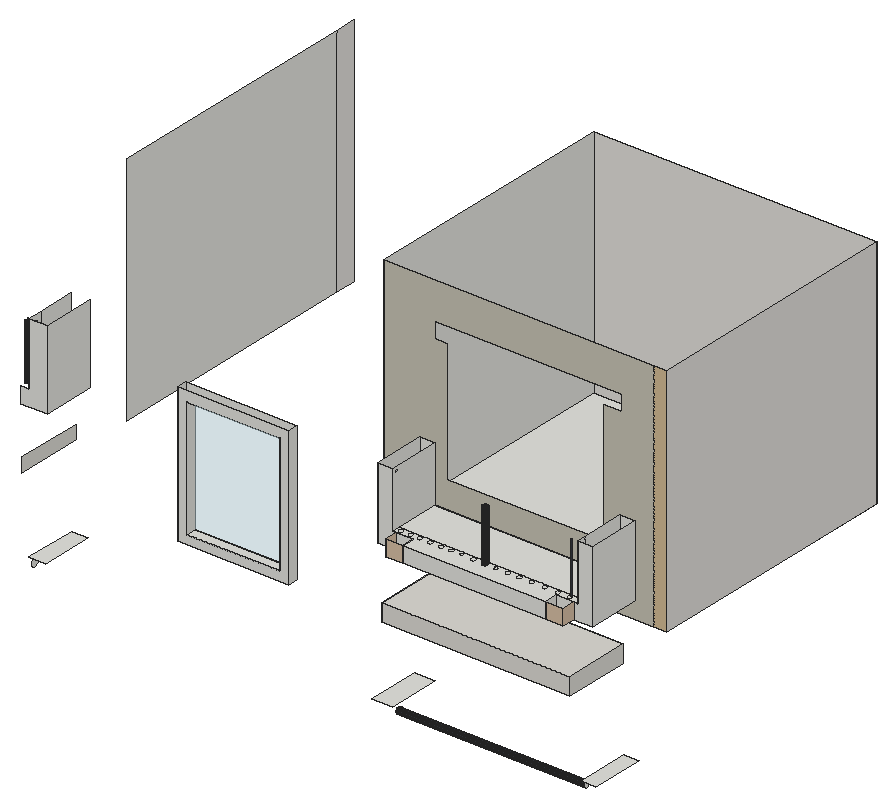
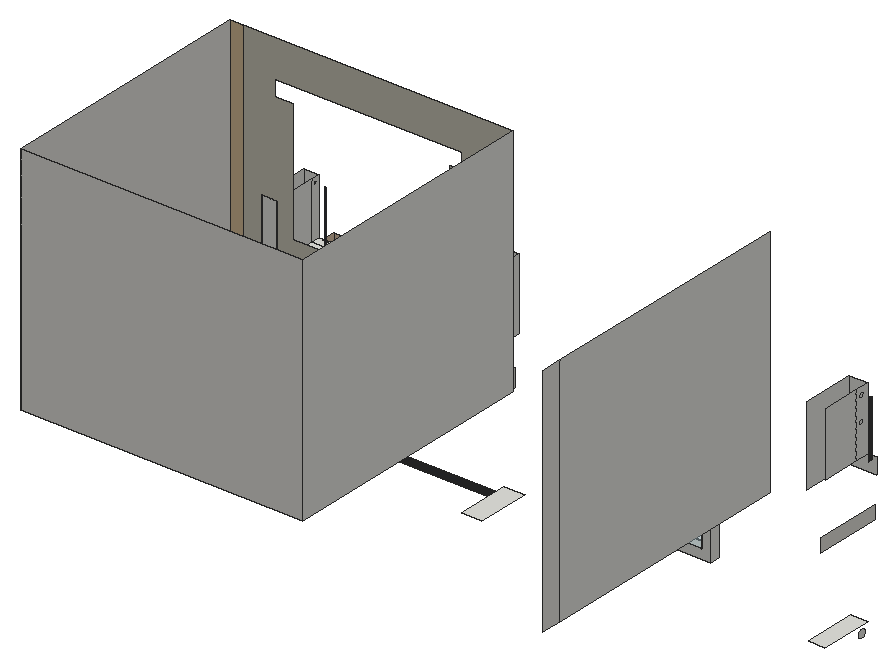
# SketchUp Ruby script. Lengths in inches.
U = 1.inch
M = Sketchup.active_model
def pt(a) = Geom::Point3d.new(a.map { |v| v * U })
def face(e, loops, mat)
  f = e.add_face(loops[0].map { |a| pt(a) })
  loops[1..].each { |l| e.add_face(l.map { |a| pt(a) }).erase! }
  f.material = f.back_material = mat if mat
  f
end
# faces: each face lists its corners as indices into pts; further lists are holes
def faces(e, pts, list, mat = nil) = list.each { |f| face(e, (f[0].is_a?(Array) ? f : [f]).map { |l| l.map { |i| pts[i] } }, mat) }
# xy, xz, yz: faces in a plane at the given z, y or x. An outline is a flat list of corners, or four numbers for a rectangle; further outlines are holes
def ring(l) = l.size == 4 ? [[l[0], l[1]], [l[2], l[1]], [l[2], l[3]], [l[0], l[3]]] : l.each_slice(2).to_a
def flat(e, list, mat, &to3) = list.each { |f| face(e, (f[0].is_a?(Array) ? f : [f]).map { |l| ring(l).map { |u, v| to3.(u, v) } }, mat) }
def xy(e, z, list, mat = nil) = flat(e, list, mat) { |x, y| [x, y, z] }
def xz(e, y, list, mat = nil) = flat(e, list, mat) { |x, z| [x, y, z] }
def yz(e, x, list, mat = nil) = flat(e, list, mat) { |y, z| [x, y, z] }
def lines(e, pts, list) = list.each { |a, b| e.add_line(pt(pts[a]), pt(pts[b])) }
# prism: a flat outline (further loops are holes) pulled along v
def prism(e, loops, v, mat = nil)
  f = face(e, loops, mat); d = Geom::Vector3d.new(v.map { |x| x * U })
  f.pushpull(f.normal.samedirection?(d) ? d.length : -d.length)
end
def box(e, o, s, mat = nil) = prism(e, [[o, [o[0] + s[0], o[1], o[2]], [o[0] + s[0], o[1] + s[1], o[2]], [o[0], o[1] + s[1], o[2]]]], [0, 0, s[2]], mat)
def at(x, y, z, deg = 0) = Geom::Transformation.translation(pt([x, y, z])) * Geom::Transformation.rotation(ORIGIN, Z_AXIS, deg.degrees)
def axes(o, x, y, z) = Geom::Transformation.new([*x, 0, *y, 0, *z, 0, *pt(o).to_a, 1])
def part(name) = M.definitions.add(name)
# library, detail: a bought-in or finely detailed component or shape, given as its bounding box
def library(name, o, s) = part(name).tap { |d| box(d.entities, o, s) }
def detail(e, o, s) = box(e.add_group.entities, o, s)
def put(e, d, t, mat = nil) = e.add_instance(d, t).tap { |i| i.material = mat if mat }
def group(e, t, mat = nil) = e.add_group.tap { |g| g.transformation = t; g.material = mat if mat }.entities
root = M.entities
M.materials.add("[Color M07]").color = [58, 58, 58]
M.materials.add("[Formica Beige]").color = [211, 187, 149]
M.materials.add("[Formica Graystone]").color = [198, 194, 180]
M.materials.add("[Formica Laminate Dark]").color = [50, 53, 60]
M.materials.add("[Formica Laminate Light]").color = [213, 189, 164]
M.materials.add("[Quartz Light Brown]").color = [199, 184, 152]
M.materials.add("[Terrazzo Tile Accent]").color = [224, 221, 217]
M.materials.add("[Terrazzo Tile Light]").color = [219, 217, 210]
M.materials.add("[Translucent Glass Safety]").color = [204, 235, 244]
M.materials["[Translucent Glass Safety]"].alpha = 0.5
xy(root,296.55,[[376.7,92.22,376.96,92.25,377.2,92.35,377.41,92.51,377.57,92.72,377.67,92.96,377.7,93.22,377.67,93.48,377.57,93.72,377.41,93.93,377.2,94.09,376.96,94.1875,376.7,94.22,376.44,94.1875,376.2,94.09,375.99,93.93,375.83,93.72,375.73,93.48,375.7,93.22,375.73,92.96,375.83,92.72,375.99,92.51,376.2,92.35,376.44,92.25]])
xy(root,296.68,[[303.57,92.22,303.83,92.25,304.07,92.35,304.28,92.51,304.44,92.72,304.54,92.96,304.57,93.22,304.54,93.48,304.44,93.72,304.28,93.93,304.07,94.09,303.83,94.1875,303.57,94.22,303.32,94.1875,303.07,94.09,302.87,93.93,302.71,93.72,302.61,93.48,302.57,93.22,302.61,92.96,302.71,92.72,302.87,92.51,303.07,92.35,303.32,92.25],[370.57,92.22,370.83,92.25,371.07,92.35,371.28,92.51,371.44,92.72,371.54,92.96,371.57,93.22,371.54,93.48,371.44,93.72,371.28,93.93,371.07,94.09,370.83,94.1875,370.57,94.22,370.32,94.1875,370.07,94.09,369.87,93.93,369.71,93.72,369.61,93.48,369.57,93.22,369.61,92.96,369.71,92.72,369.87,92.51,370.07,92.35,370.32,92.25]])
xy(root,296.93,[[352.2,92.22,352.46,92.25,352.7,92.35,352.91,92.51,353.07,92.72,353.17,92.96,353.2,93.22,353.17,93.48,353.07,93.72,352.91,93.93,352.7,94.09,352.46,94.1875,352.2,94.22,351.94,94.1875,351.7,94.09,351.49,93.93,351.33,93.72,351.23,93.48,351.2,93.22,351.23,92.96,351.33,92.72,351.49,92.51,351.7,92.35,351.94,92.25]])
xy(root,297.05,[[298.07,92.22,298.33,92.25,298.57,92.35,298.78,92.51,298.94,92.72,299.04,92.96,299.07,93.22,299.04,93.48,298.94,93.72,298.78,93.93,298.57,94.09,298.33,94.1875,298.07,94.22,297.82,94.1875,297.57,94.09,297.37,93.93,297.21,93.72,297.11,93.48,297.07,93.22,297.11,92.96,297.21,92.72,297.37,92.51,297.57,92.35,297.82,92.25],[323.57,92.22,323.83,92.25,324.07,92.35,324.28,92.51,324.44,92.72,324.54,92.96,324.57,93.22,324.54,93.48,324.44,93.72,324.28,93.93,324.07,94.09,323.83,94.1875,323.57,94.22,323.32,94.1875,323.07,94.09,322.87,93.93,322.71,93.72,322.61,93.48,322.57,93.22,322.61,92.96,322.71,92.72,322.87,92.51,323.07,92.35,323.32,92.25]])
xy(root,297.11,[[337.23,91.64,337.68,91.7,338.11,91.875,338.47,92.15,338.75,92.51,338.92,92.9375,338.98,93.39,338.92,93.84,338.75,94.26,338.47,94.625,338.11,94.9,337.68,95.08,337.23,95.14,336.78,95.08,336.36,94.9,335.99,94.625,335.72,94.26,335.54,93.84,335.48,93.39,335.54,92.9375,335.72,92.51,335.99,92.15,336.36,91.875,336.78,91.7]],"[Formica Laminate Dark]")
xy(root,297.18,[[329.95,92.22,330.21,92.25,330.45,92.35,330.66,92.51,330.82,92.72,330.92,92.96,330.95,93.22,330.92,93.48,330.82,93.72,330.66,93.93,330.45,94.09,330.21,94.1875,329.95,94.22,329.69,94.1875,329.45,94.09,329.24,93.93,329.08,93.72,328.98,93.48,328.95,93.22,328.98,92.96,329.08,92.72,329.24,92.51,329.45,92.35,329.69,92.25]])
xy(root,297.44,[[316.7,92.22,316.96,92.25,317.2,92.35,317.41,92.51,317.57,92.72,317.67,92.96,317.7,93.22,317.67,93.48,317.57,93.72,317.41,93.93,317.2,94.09,316.96,94.1875,316.7,94.22,316.44,94.1875,316.2,94.09,315.99,93.93,315.83,93.72,315.73,93.48,315.7,93.22,315.73,92.96,315.83,92.72,315.99,92.51,316.2,92.35,316.44,92.25]])
xy(root,297.55,[[345.7,92.22,345.96,92.25,346.2,92.35,346.41,92.51,346.57,92.72,346.67,92.96,346.7,93.22,346.67,93.48,346.57,93.72,346.41,93.93,346.2,94.09,345.96,94.1875,345.7,94.22,345.44,94.1875,345.2,94.09,344.99,93.93,344.83,93.72,344.73,93.48,344.7,93.22,344.73,92.96,344.83,92.72,344.99,92.51,345.2,92.35,345.44,92.25]])
xy(root,297.74,[[310.2,92.22,310.46,92.25,310.7,92.35,310.91,92.51,311.07,92.72,311.17,92.96,311.2,93.22,311.17,93.48,311.07,93.72,310.91,93.93,310.7,94.09,310.55,94.15,309.85,94.15,309.7,94.09,309.49,93.93,309.33,93.72,309.23,93.48,309.2,93.22,309.23,92.96,309.33,92.72,309.49,92.51,309.7,92.35,309.94,92.25],[358.14,92.22,358.4,92.25,358.64,92.35,358.84,92.51,359,92.72,359.1,92.96,359.14,93.22,359.1,93.48,359,93.72,358.84,93.93,358.64,94.09,358.49,94.15,357.78,94.15,357.64,94.09,357.43,93.93,357.27,93.72,357.17,93.48,357.14,93.22,357.17,92.96,357.27,92.72,357.43,92.51,357.64,92.35,357.88,92.25],[364.2,92.22,364.46,92.25,364.7,92.35,364.91,92.51,365.07,92.72,365.17,92.96,365.2,93.22,365.17,93.48,365.07,93.72,364.91,93.93,364.7,94.09,364.46,94.1875,364.2,94.22,363.94,94.1875,363.7,94.09,363.49,93.93,363.33,93.72,363.23,93.48,363.2,93.22,363.23,92.96,363.33,92.72,363.49,92.51,363.7,92.35,363.94,92.25],[309.85,94.15,310.55,94.15,310.46,94.1875,310.2,94.22,309.94,94.1875],[357.78,94.15,358.49,94.15,358.4,94.1875,358.14,94.22,357.88,94.1875]])
xy(root,299.8,[[284.91,89.73,294.34,114.1],[381.41,89.73,388.23,114.1]])
xy(root,302.83,[[126.66,89.73,134.24,114.1]])
xy(root,319.3125,[[179.41,109.54,230.79,114.1]])
xy(root,323.67,[[183.77,109.54,226.43,114.1]])
xy(root,334.91,[[299.6,103.17,374.79,114.1]],"[Quartz Light Brown]")
xy(root,336.3125,[[299.6,105.17,374.79,114.1]])
xy(root,336.3125,[[299.6,103.17,374.79,105.17]],"[Quartz Light Brown]")
xy(root,337.71,[[299.6,105.17,374.79,114.1]])
xy(root,337.71,[[[294.42,83.29,294.42,114.1,299.6,114.1,299.6,105.17,374.79,105.17,374.79,114.1,381.23,114.1,381.23,83.29],[374.29,84.01,374.87,84.08,375.41,84.31,375.88,84.67,376.24,85.13,376.46,85.67,376.54,86.26,376.46,86.84,376.24,87.38,375.88,87.85,375.41,88.21,374.87,88.43,374.29,88.51,373.71,88.43,373.16,88.21,372.7,87.85,372.34,87.38,372.12,86.84,372.04,86.26,372.12,85.67,372.34,85.13,372.7,84.67,373.16,84.31,373.71,84.08],[302.73,84.01,303.31,84.08,303.85,84.31,304.32,84.67,304.67,85.13,304.9,85.67,304.98,86.26,304.9,86.84,304.67,87.38,304.32,87.85,303.85,88.21,303.31,88.43,302.73,88.51,302.14,88.43,301.6,88.21,301.14,87.85,300.78,87.38,300.55,86.84,300.48,86.26,300.55,85.67,300.78,85.13,301.14,84.67,301.6,84.31,302.14,84.08]]],"[Terrazzo Tile Light]")
xy(root,345.83,[[294.42,83.29,381.23,114.1]],"[Terrazzo Tile Light]")
xy(root,357.6875,[[270.97,114.1,401.16,235.11]])
xy(root,365.35,[[303.82,83.54,303.82,89.73,287.58,89.73,287.58,114.1,386.54,114.1,386.54,89.73,369.85,89.73,369.85,83.54]])
xy(root,365.35,[[295.97,83.54,303.82,89.73],[369.85,83.54,377.7,89.73]],"[Formica Laminate Light]")
xy(root,372.6,[[[303.82,83.54,369.85,83.54,369.85,89.73,379.76,89.73,379.76,93.62,294.32,93.62,294.32,89.73,303.82,89.73],[335.44,90.49,335.13,90.53,334.85,90.64,334.6,90.83,334.41,91.08,334.29,91.37,334.25,91.67,334.29,91.98,334.41,92.27,334.6,92.51,334.85,92.7,335.13,92.82,335.44,92.86,335.75,92.82,336.03,92.7,336.28,92.51,336.47,92.27,336.59,91.98,336.63,91.67,336.59,91.37,336.47,91.08,336.28,90.83,336.03,90.64,335.75,90.53],[340.51,90.87,340.3,90.9,340.1,90.98,339.9375,91.11,339.81,91.28,339.73,91.47,339.7,91.68,339.73,91.89,339.81,92.09,339.9375,92.26,340.1,92.39,340.3,92.47,340.51,92.5,340.72,92.47,340.92,92.39,341.09,92.26,341.21,92.09,341.3,91.89,341.32,91.68,341.3,91.47,341.21,91.28,341.09,91.11,340.92,90.98,340.72,90.9],[374.64,90.87,374.43,90.9,374.23,90.98,374.0625,91.11,373.93,91.28,373.85,91.47,373.82,91.68,373.85,91.89,373.93,92.09,374.0625,92.26,374.23,92.39,374.43,92.47,374.64,92.5,374.85,92.47,375.04,92.39,375.21,92.26,375.34,92.09,375.42,91.89,375.45,91.68,375.42,91.47,375.34,91.28,375.21,91.11,375.04,90.98,374.85,90.9],[345.89,90.87,345.68,90.9,345.48,90.98,345.3125,91.11,345.18,91.28,345.1,91.47,345.07,91.68,345.1,91.89,345.18,92.09,345.3125,92.26,345.48,92.39,345.68,92.47,345.89,92.5,346.1,92.47,346.29,92.39,346.46,92.26,346.59,92.09,346.67,91.89,346.7,91.68,346.67,91.47,346.59,91.28,346.46,91.11,346.29,90.98,346.1,90.9],[369.07,90.87,368.86,90.9,368.67,90.98,368.5,91.11,368.37,91.28,368.29,91.47,368.26,91.68,368.29,91.89,368.37,92.09,368.5,92.26,368.67,92.39,368.86,92.47,369.07,92.5,369.28,92.47,369.48,92.39,369.65,92.26,369.78,92.09,369.86,91.89,369.89,91.68,369.86,91.47,369.78,91.28,369.65,91.11,369.48,90.98,369.28,90.9],[351.2,90.87,350.99,90.9,350.79,90.98,350.625,91.11,350.49,91.28,350.41,91.47,350.39,91.68,350.41,91.89,350.49,92.09,350.625,92.26,350.79,92.39,350.99,92.47,351.2,92.5,351.41,92.47,351.6,92.39,351.77,92.26,351.9,92.09,351.98,91.89,352.01,91.68,351.98,91.47,351.9,91.28,351.77,91.11,351.6,90.98,351.41,90.9],[363.01,90.87,362.8,90.9,362.6,90.98,362.4375,91.11,362.31,91.28,362.23,91.47,362.2,91.68,362.23,91.89,362.31,92.09,362.4375,92.26,362.6,92.39,362.8,92.47,363.01,92.5,363.22,92.47,363.42,92.39,363.59,92.26,363.71,92.09,363.8,91.89,363.82,91.68,363.8,91.47,363.71,91.28,363.59,91.11,363.42,90.98,363.22,90.9],[356.89,90.87,356.68,90.9,356.48,90.98,356.3125,91.11,356.18,91.28,356.1,91.47,356.07,91.68,356.1,91.89,356.18,92.09,356.3125,92.26,356.48,92.39,356.68,92.47,356.89,92.5,357.1,92.47,357.29,92.39,357.46,92.26,357.59,92.09,357.67,91.89,357.7,91.68,357.67,91.47,357.59,91.28,357.46,91.11,357.29,90.98,357.1,90.9],[296.64,90.87,296.43,90.9,296.23,90.98,296.0625,91.11,295.93,91.28,295.85,91.47,295.82,91.68,295.85,91.89,295.93,92.09,296.0625,92.26,296.23,92.39,296.43,92.47,296.64,92.5,296.85,92.47,297.04,92.39,297.21,92.26,297.34,92.09,297.42,91.89,297.45,91.68,297.42,91.47,297.34,91.28,297.21,91.11,297.04,90.98,296.85,90.9],[301.07,90.87,300.86,90.9,300.67,90.98,300.5,91.11,300.37,91.28,300.29,91.47,300.26,91.68,300.29,91.89,300.37,92.09,300.5,92.26,300.67,92.39,300.86,92.47,301.07,92.5,301.28,92.47,301.48,92.39,301.65,92.26,301.78,92.09,301.86,91.89,301.89,91.68,301.86,91.47,301.78,91.28,301.65,91.11,301.48,90.98,301.28,90.9],[305.39,90.87,305.18,90.9,304.98,90.98,304.8125,91.11,304.68,91.28,304.6,91.47,304.57,91.68,304.6,91.89,304.68,92.09,304.8125,92.26,304.98,92.39,305.18,92.47,305.39,92.5,305.6,92.47,305.79,92.39,305.96,92.26,306.09,92.09,306.17,91.89,306.2,91.68,306.17,91.47,306.09,91.28,305.96,91.11,305.79,90.98,305.6,90.9],[310.2,90.87,309.99,90.9,309.79,90.98,309.625,91.11,309.49,91.28,309.41,91.47,309.39,91.68,309.41,91.89,309.49,92.09,309.625,92.26,309.79,92.39,309.99,92.47,310.2,92.5,310.41,92.47,310.6,92.39,310.77,92.26,310.9,92.09,310.98,91.89,311.01,91.68,310.98,91.47,310.9,91.28,310.77,91.11,310.6,90.98,310.41,90.9],[315.2,90.87,314.99,90.9,314.79,90.98,314.625,91.11,314.49,91.28,314.41,91.47,314.39,91.68,314.41,91.89,314.49,92.09,314.625,92.26,314.79,92.39,314.99,92.47,315.2,92.5,315.41,92.47,315.6,92.39,315.77,92.26,315.9,92.09,315.98,91.89,316.01,91.68,315.98,91.47,315.9,91.28,315.77,91.11,315.6,90.98,315.41,90.9],[330.07,90.87,329.86,90.9,329.67,90.98,329.5,91.11,329.37,91.28,329.29,91.47,329.26,91.68,329.29,91.89,329.37,92.09,329.5,92.26,329.67,92.39,329.86,92.47,330.07,92.5,330.28,92.47,330.48,92.39,330.65,92.26,330.78,92.09,330.86,91.89,330.89,91.68,330.86,91.47,330.78,91.28,330.65,91.11,330.48,90.98,330.28,90.9],[324.82,90.87,324.61,90.9,324.42,90.98,324.25,91.11,324.12,91.28,324.04,91.47,324.01,91.68,324.04,91.89,324.12,92.09,324.25,92.26,324.42,92.39,324.61,92.47,324.82,92.5,325.03,92.47,325.23,92.39,325.4,92.26,325.53,92.09,325.61,91.89,325.64,91.68,325.61,91.47,325.53,91.28,325.4,91.11,325.23,90.98,325.03,90.9],[319.89,90.87,319.68,90.9,319.48,90.98,319.3125,91.11,319.18,91.28,319.1,91.47,319.07,91.68,319.1,91.89,319.18,92.09,319.3125,92.26,319.48,92.39,319.68,92.47,319.89,92.5,320.1,92.47,320.29,92.39,320.46,92.26,320.59,92.09,320.67,91.89,320.7,91.68,320.67,91.47,320.59,91.28,320.46,91.11,320.29,90.98,320.1,90.9]],[335.44,90.49,335.13,90.53,334.85,90.64,334.6,90.83,334.41,91.08,334.29,91.37,334.25,91.67,334.29,91.98,334.41,92.27,334.6,92.51,334.85,92.7,335.13,92.82,335.44,92.86,335.75,92.82,336.03,92.7,336.28,92.51,336.47,92.27,336.59,91.98,336.63,91.67,336.59,91.37,336.47,91.08,336.28,90.83,336.03,90.64,335.75,90.53],[296.64,90.87,296.43,90.9,296.23,90.98,296.0625,91.11,295.93,91.28,295.85,91.47,295.82,91.68,295.85,91.89,295.93,92.09,296.0625,92.26,296.23,92.39,296.43,92.47,296.64,92.5,296.85,92.47,297.04,92.39,297.21,92.26,297.34,92.09,297.42,91.89,297.45,91.68,297.42,91.47,297.34,91.28,297.21,91.11,297.04,90.98,296.85,90.9],[301.07,90.87,300.86,90.9,300.67,90.98,300.5,91.11,300.37,91.28,300.29,91.47,300.26,91.68,300.29,91.89,300.37,92.09,300.5,92.26,300.67,92.39,300.86,92.47,301.07,92.5,301.28,92.47,301.48,92.39,301.65,92.26,301.78,92.09,301.86,91.89,301.89,91.68,301.86,91.47,301.78,91.28,301.65,91.11,301.48,90.98,301.28,90.9],[305.39,90.87,305.18,90.9,304.98,90.98,304.8125,91.11,304.68,91.28,304.6,91.47,304.57,91.68,304.6,91.89,304.68,92.09,304.8125,92.26,304.98,92.39,305.18,92.47,305.39,92.5,305.6,92.47,305.79,92.39,305.96,92.26,306.09,92.09,306.17,91.89,306.2,91.68,306.17,91.47,306.09,91.28,305.96,91.11,305.79,90.98,305.6,90.9],
  [310.2,90.87,309.99,90.9,309.79,90.98,309.625,91.11,309.49,91.28,309.41,91.47,309.39,91.68,309.41,91.89,309.49,92.09,309.625,92.26,309.79,92.39,309.99,92.47,310.2,92.5,310.41,92.47,310.6,92.39,310.77,92.26,310.9,92.09,310.98,91.89,311.01,91.68,310.98,91.47,310.9,91.28,310.77,91.11,310.6,90.98,310.41,90.9],[315.2,90.87,314.99,90.9,314.79,90.98,314.625,91.11,314.49,91.28,314.41,91.47,314.39,91.68,314.41,91.89,314.49,92.09,314.625,92.26,314.79,92.39,314.99,92.47,315.2,92.5,315.41,92.47,315.6,92.39,315.77,92.26,315.9,92.09,315.98,91.89,316.01,91.68,315.98,91.47,315.9,91.28,315.77,91.11,315.6,90.98,315.41,90.9],[319.89,90.87,319.68,90.9,319.48,90.98,319.3125,91.11,319.18,91.28,319.1,91.47,319.07,91.68,319.1,91.89,319.18,92.09,319.3125,92.26,319.48,92.39,319.68,92.47,319.89,92.5,320.1,92.47,320.29,92.39,320.46,92.26,320.59,92.09,320.67,91.89,320.7,91.68,320.67,91.47,320.59,91.28,320.46,91.11,320.29,90.98,320.1,90.9],[324.82,90.87,324.61,90.9,324.42,90.98,324.25,91.11,324.12,91.28,324.04,91.47,324.01,91.68,324.04,91.89,324.12,92.09,324.25,92.26,324.42,92.39,324.61,92.47,324.82,92.5,325.03,92.47,325.23,92.39,325.4,92.26,325.53,92.09,325.61,91.89,325.64,91.68,325.61,91.47,325.53,91.28,325.4,91.11,325.23,90.98,325.03,90.9],[330.07,90.87,329.86,90.9,329.67,90.98,329.5,91.11,329.37,91.28,329.29,91.47,329.26,91.68,329.29,91.89,329.37,92.09,329.5,92.26,329.67,92.39,329.86,92.47,330.07,92.5,330.28,92.47,330.48,92.39,330.65,92.26,330.78,92.09,330.86,91.89,330.89,91.68,330.86,91.47,330.78,91.28,330.65,91.11,330.48,90.98,330.28,90.9],
  [340.51,90.87,340.3,90.9,340.1,90.98,339.9375,91.11,339.81,91.28,339.73,91.47,339.7,91.68,339.73,91.89,339.81,92.09,339.9375,92.26,340.1,92.39,340.3,92.47,340.51,92.5,340.72,92.47,340.92,92.39,341.09,92.26,341.21,92.09,341.3,91.89,341.32,91.68,341.3,91.47,341.21,91.28,341.09,91.11,340.92,90.98,340.72,90.9],[345.89,90.87,345.68,90.9,345.48,90.98,345.3125,91.11,345.18,91.28,345.1,91.47,345.07,91.68,345.1,91.89,345.18,92.09,345.3125,92.26,345.48,92.39,345.68,92.47,345.89,92.5,346.1,92.47,346.29,92.39,346.46,92.26,346.59,92.09,346.67,91.89,346.7,91.68,346.67,91.47,346.59,91.28,346.46,91.11,346.29,90.98,346.1,90.9],[351.2,90.87,350.99,90.9,350.79,90.98,350.625,91.11,350.49,91.28,350.41,91.47,350.39,91.68,350.41,91.89,350.49,92.09,350.625,92.26,350.79,92.39,350.99,92.47,351.2,92.5,351.41,92.47,351.6,92.39,351.77,92.26,351.9,92.09,351.98,91.89,352.01,91.68,351.98,91.47,351.9,91.28,351.77,91.11,351.6,90.98,351.41,90.9],[356.89,90.87,356.68,90.9,356.48,90.98,356.3125,91.11,356.18,91.28,356.1,91.47,356.07,91.68,356.1,91.89,356.18,92.09,356.3125,92.26,356.48,92.39,356.68,92.47,356.89,92.5,357.1,92.47,357.29,92.39,357.46,92.26,357.59,92.09,357.67,91.89,357.7,91.68,357.67,91.47,357.59,91.28,357.46,91.11,357.29,90.98,357.1,90.9],[363.01,90.87,362.8,90.9,362.6,90.98,362.4375,91.11,362.31,91.28,362.23,91.47,362.2,91.68,362.23,91.89,362.31,92.09,362.4375,92.26,362.6,92.39,362.8,92.47,363.01,92.5,363.22,92.47,363.42,92.39,363.59,92.26,363.71,92.09,363.8,91.89,363.82,91.68,363.8,91.47,363.71,91.28,363.59,91.11,363.42,90.98,363.22,90.9],
  [369.07,90.87,368.86,90.9,368.67,90.98,368.5,91.11,368.37,91.28,368.29,91.47,368.26,91.68,368.29,91.89,368.37,92.09,368.5,92.26,368.67,92.39,368.86,92.47,369.07,92.5,369.28,92.47,369.48,92.39,369.65,92.26,369.78,92.09,369.86,91.89,369.89,91.68,369.86,91.47,369.78,91.28,369.65,91.11,369.48,90.98,369.28,90.9],[374.64,90.87,374.43,90.9,374.23,90.98,374.0625,91.11,373.93,91.28,373.85,91.47,373.82,91.68,373.85,91.89,373.93,92.09,374.0625,92.26,374.23,92.39,374.43,92.47,374.64,92.5,374.85,92.47,375.04,92.39,375.21,92.26,375.34,92.09,375.42,91.89,375.45,91.68,375.42,91.47,375.34,91.28,375.21,91.11,375.04,90.98,374.85,90.9],[294.32,93.62,379.76,114.1]])
xz(root,83.29,[[294.42,337.71,381.23,345.83]],"[Terrazzo Tile Light]")
xz(root,83.54,[[303.82,365.35,369.85,372.6]])
xz(root,83.54,[[295.97,365.35,303.82,372.6],[369.85,365.35,377.7,372.6]],"[Formica Laminate Light]")
xz(root,89.73,[[122.61,365.02,135.17,365.02,135.17,401.52,126.56,401.52,126.56,372.27,122.61,372.27],[287.58,365.35,295.97,365.35,295.97,372.6,294.32,372.6,294.32,398.47,287.58,398.47],[295.97,365.35,303.82,372.6],[369.85,365.35,377.7,372.6],[377.7,365.35,386.54,365.35,386.54,398.47,379.76,398.47,379.76,372.6,377.7,372.6]])
xz(root,103.17,[[299.6,334.91,374.79,336.3125]],"[Quartz Light Brown]")
xz(root,105.17,[[299.6,336.3125,374.79,337.71]],"[Quartz Light Brown]")
xz(root,109.54,[[[179.41,319.3125,230.79,383],[183.77,323.67,226.43,378.64]]])
xz(root,114.1,[[[179.41,319.3125,230.79,383],[183.77,323.67,226.43,378.64]],[299.6,334.91,374.79,336.3125],[299.6,336.3125,374.79,337.71],[294.42,337.71,381.23,345.83],[287.58,365.35,287.58,398.47,294.32,398.47,294.32,372.6,379.76,372.6,379.76,398.47,386.54,398.47,386.54,365.35]])
xz(root,114.1,[[395.49,357.6875,401.16,465.6875]],"[Formica Beige]")
xz(root,114.1,[[[270.97,357.6875,395.49,465.6875],[299.92,385.12,299.92,441.22,294.2,441.22,294.2,448.85,380.45,448.85,380.45,441.22,372.17,441.22,372.17,385.12],[287.58,365.35,287.58,398.47,294.32,398.47,294.32,372.6,379.76,372.6,379.76,398.47,386.54,398.47,386.54,365.35]]],"[Formica Graystone]")
xz(root,114.1,[[183.77,323.67,226.43,378.64]],"[Translucent Glass Safety]")
xz(root,235.11,[[270.97,357.6875,401.16,465.6875]],"[Terrazzo Tile Accent]")
yz(root,126.56,[[[89.73,372.27,96.33,401.52],[93.49,396.95,93.81,396.99,94.11,397.12,94.37,397.32,94.57,397.58,94.69,397.88,94.74,398.2,94.69,398.52,94.57,398.83,94.37,399.09,94.11,399.28,93.81,399.41,93.49,399.45,93.16,399.41,92.86,399.28,92.6,399.09,92.4,398.83,92.28,398.52,92.24,398.2,92.28,397.88,92.4,397.58,92.6,397.32,92.86,397.12,93.16,396.99],[93.62,385.75,93.93,385.79,94.21,385.91,94.46,386.1,94.65,386.34,94.77,386.63,94.81,386.9375,94.77,387.25,94.65,387.53,94.46,387.78,94.21,387.97,93.93,388.09,93.62,388.125,93.3125,388.09,93.03,387.97,92.78,387.78,92.59,387.53,92.47,387.25,92.43,386.9375,92.47,386.63,92.59,386.34,92.78,386.1,93.03,385.91,93.3125,385.79]],[96.33,372.27,114.1,401.52]])
yz(root,126.66,[[92.96,297.54,93.42,297.6,93.84,297.77,94.2,298.05,94.48,298.41,94.65,298.84,94.71,299.29,94.65,299.74,94.48,300.16,94.2,300.53,93.84,300.8,93.42,300.98,92.96,301.04,92.51,300.98,92.09,300.8,91.73,300.53,91.45,300.16,91.27,299.74,91.21,299.29,91.27,298.84,91.45,298.41,91.73,298.05,92.09,297.77,92.51,297.6]])
yz(root,128.55,[[83.35,341.31,114.1,347.68]],"[Terrazzo Tile Light]")
yz(root,135.17,[[89.73,365.02,114.1,401.52]])
yz(root,152.39,[[114.1,357.6875,235.11,465.6875]])
yz(root,152.39,[[235.11,357.6875,244.83,465.6875]],"[Terrazzo Tile Accent]")
yz(root,179.41,[[109.54,319.3125,114.1,383]])
yz(root,183.77,[[109.54,323.67,114.1,378.64]])
yz(root,226.43,[[109.54,323.67,114.1,378.64]])
yz(root,230.79,[[109.54,319.3125,114.1,383]])
yz(root,270.97,[[114.1,357.6875,235.11,465.6875]])
yz(root,287.58,[[89.73,365.35,114.1,398.47]])
yz(root,294.32,[[[89.73,372.6,114.1,398.47],[91.8125,395.54,91.6,395.57,91.41,395.65,91.24,395.78,91.11,395.95,91.03,396.14,91,396.35,91.03,396.5625,91.11,396.76,91.24,396.93,91.41,397.06,91.6,397.14,91.8125,397.16,92.02,397.14,92.22,397.06,92.39,396.93,92.52,396.76,92.6,396.5625,92.625,396.35,92.6,396.14,92.52,395.95,92.39,395.78,92.22,395.65,92.02,395.57]]])
yz(root,294.42,[[83.29,337.71,114.1,345.83]],"[Terrazzo Tile Light]")
yz(root,295.97,[[83.54,365.35,89.73,372.6]],"[Formica Laminate Light]")
yz(root,299.6,[[103.17,334.91,114.1,336.3125],[105.17,336.3125,114.1,337.71]],"[Quartz Light Brown]")
yz(root,303.82,[[83.54,365.35,89.73,372.6]])
yz(root,369.85,[[83.54,365.35,89.73,372.6]])
yz(root,374.79,[[103.17,334.91,114.1,336.3125],[105.17,336.3125,114.1,337.71]],"[Quartz Light Brown]")
yz(root,377.7,[[83.54,365.35,89.73,372.6]],"[Formica Laminate Light]")
yz(root,379.76,[[[89.73,372.6,93.62,398.47],[91.8125,395.54,92.02,395.57,92.22,395.65,92.39,395.78,92.52,395.95,92.6,396.14,92.625,396.35,92.6,396.5625,92.52,396.76,92.39,396.93,92.22,397.06,92.02,397.14,91.8125,397.16,91.6,397.14,91.41,397.06,91.24,396.93,91.11,396.76,91.03,396.5625,91,396.35,91.03,396.14,91.11,395.95,91.24,395.78,91.41,395.65,91.6,395.57]],[93.62,372.6,114.1,398.47]])
yz(root,381.23,[[83.29,337.71,114.1,345.83]],"[Terrazzo Tile Light]")
yz(root,381.41,[[93.0625,295.87,93.39,295.91,93.6875,296.04,93.95,296.23,94.15,296.49,94.27,296.79,94.3125,297.12,94.27,297.44,94.15,297.74,93.95,298,93.6875,298.2,93.39,298.33,93.0625,298.37,92.74,298.33,92.4375,298.2,92.18,298,91.98,297.74,91.86,297.44,91.8125,297.12,91.86,296.79,91.98,296.49,92.18,296.23,92.4375,296.04,92.74,295.91]])
yz(root,386.54,[[89.73,365.35,114.1,398.47]])
yz(root,401.16,[[114.1,357.6875,235.11,465.6875]],"[Terrazzo Tile Accent]")
p = [[381.41,92.74,295.91],[381.41,92.4375,296.04],[294.34,92.4375,296.04],[294.34,92.74,295.91],[381.41,93.0625,295.87],[294.34,93.0625,295.87],
  [381.41,93.39,295.91],[294.34,93.39,295.91],[381.41,93.6875,296.04],[294.34,93.6875,296.04],[381.41,92.18,296.23],[294.34,92.18,296.23],
  [381.41,93.95,296.23],[294.34,93.95,296.23],[381.41,91.98,296.49],[294.34,91.98,296.49],[381.41,94.15,296.49],[294.34,94.15,296.49],
  [381.41,91.86,296.79],[294.34,91.86,296.79],[381.41,94.27,296.79],[294.34,94.27,296.79],[381.41,91.8125,297.12],[294.34,91.8125,297.12],
  [381.41,94.3125,297.12],[294.34,94.3125,297.12],[381.41,91.86,297.44],[294.34,91.86,297.44],[381.41,94.27,297.44],[294.34,94.27,297.44],
  [381.41,91.98,297.74],[294.34,91.98,297.74],[381.41,94.15,297.74],[294.34,94.15,297.74],[309.85,94.15,297.74],[310.55,94.15,297.74],
  [357.78,94.15,297.74],[358.49,94.15,297.74],[381.41,92.18,298],[294.34,92.18,298],[381.41,93.95,298],[294.34,93.95,298],
  [381.41,92.4375,298.2],[294.34,92.4375,298.2],[381.41,93.6875,298.2],[294.34,93.6875,298.2],[381.41,92.74,298.33],[294.34,92.74,298.33],
  [381.41,93.39,298.33],[294.34,93.39,298.33],[381.41,93.0625,298.37],[294.34,93.0625,298.37],[122.71,92.2,372.27],[122.92,92.35,372.27],
  [122.92,92.35,398.4],[122.71,92.2,398.4],[123.08,92.5625,372.27],[123.08,92.5625,398.4],[123.18,92.8,372.27],[123.18,92.8,398.4],
  [123.21,93.0625,372.27],[123.21,93.0625,398.4],[123.18,93.32,372.27],[123.18,93.32,398.4],[123.08,93.5625,372.27],[123.08,93.5625,398.4],
  [122.92,93.77,372.27],[122.92,93.77,398.4],[122.71,93.93,372.27],[122.71,93.93,385.79],[122.71,93.93,388.09],[122.71,93.93,398.4],
  [122.47,94.03,372.27],[122.47,94.03,398.4],[334.85,90.64,372.6],[335.13,90.53,372.6],[335.13,90.53,396.5625],[334.85,90.64,396.5625],
  [335.44,90.49,372.6],[335.44,90.49,396.5625],[335.75,90.53,372.6],[335.75,90.53,396.5625],[336.03,90.64,372.6],[336.03,90.64,396.5625],
  [334.6,90.83,372.6],[334.6,90.83,396.5625],[336.28,90.83,372.6],[336.28,90.83,396.5625],[334.41,91.08,372.6],[334.45,91.03,396.5625],
  [334.41,91.08,396.5625],[336.47,91.08,372.6],[336.47,91.08,396.5625],[336.43,91.03,396.5625],[334.29,91.37,372.6],[334.29,91.37,396.5625],
  [336.59,91.37,372.6],[336.59,91.37,396.5625],[334.25,91.67,372.6],[334.25,91.67,396.5625],[336.63,91.67,372.6],[336.63,91.67,396.5625],
  [334.29,91.98,372.6],[334.29,91.98,396.5625],[336.59,91.98,372.6],[336.59,91.98,396.5625],[334.41,92.27,372.6],[334.41,92.27,396.5625],
  [336.47,92.27,372.6],[336.47,92.27,396.5625],[334.6,92.51,372.6],[334.6,92.51,396.5625],[336.28,92.51,372.6],[336.28,92.51,396.5625],
  [375.04,92.39,372.6],[374.85,92.47,372.6],[374.85,92.47,396.41],[375.04,92.39,396.41],[375.04,92.39,395.78],[334.85,92.7,372.6],
  [334.71,92.6,396.5625],[334.85,92.7,396.5625],[336.03,92.7,372.6],[336.03,92.7,396.5625],[336.17,92.6,396.5625],[374.64,92.5,372.6],
  [374.43,92.47,372.6],[374.43,92.47,396.41],[374.64,92.5,396.41],[335.13,92.82,372.6],[335.13,92.82,396.5625],[335.75,92.82,372.6],
  [335.75,92.82,396.5625],[335.44,92.86,372.6],[335.44,92.86,396.5625]]
faces(root,p,[[0,1,2,3],[4,0,3,5],[6,4,5,7],[8,6,7,9],[1,10,11,2],[12,8,9,13],[10,14,15,11],[16,12,13,17],
  [14,18,19,15],[20,16,17,21],[18,22,23,19],[24,20,21,25],[22,26,27,23],[28,24,25,29],[26,30,31,27],[32,28,29,33,34,35,36,37],
  [30,38,39,31],[40,32,37,36,35,34,33,41],[38,42,43,39],[44,40,41,45],[42,46,47,43],[48,44,45,49],[46,50,51,47],[50,48,49,51],
  [74,75,76,77],[75,78,79,76],[78,80,81,79],[80,82,83,81],[84,74,77,85],[82,86,87,83],[88,84,85,89,90],[86,91,92,93,87],
  [94,88,90,95],[91,96,97,92],[98,94,95,99],[96,100,101,97],[102,98,99,103],[100,104,105,101],[106,102,103,107],[104,108,109,105],
  [110,106,107,111],[108,112,113,109],[114,115,116,117,118],[119,110,111,120,121],[112,122,123,124,113],[125,126,127,128],[115,125,128,116],[129,119,121,130],
  [122,131,132,123],[133,129,130,134],[131,133,134,132]],"[Formica Laminate Dark]")
faces(root,p,[[52,53,54,55],[53,56,57,54],[56,58,59,57],[58,60,61,59],[60,62,63,61],[62,64,65,63],[64,66,67,65],[66,68,69,70,71,67],
  [68,72,73,71,70,69]],"[Color M07]")
